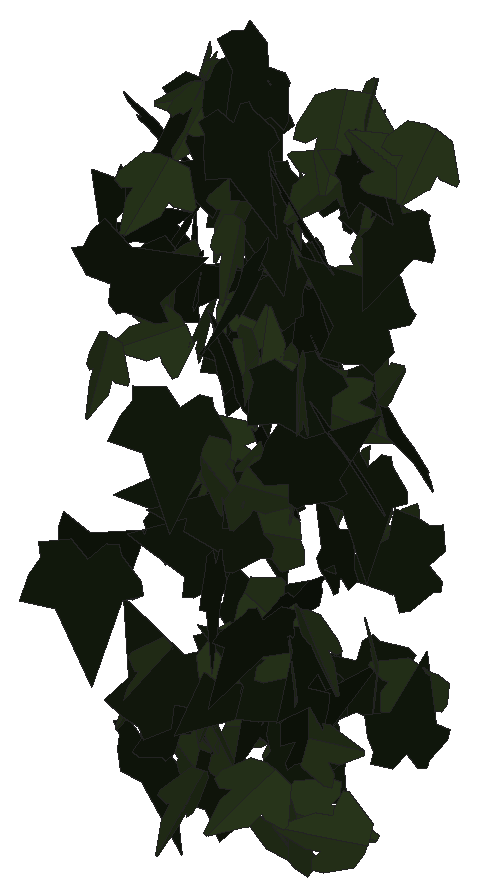
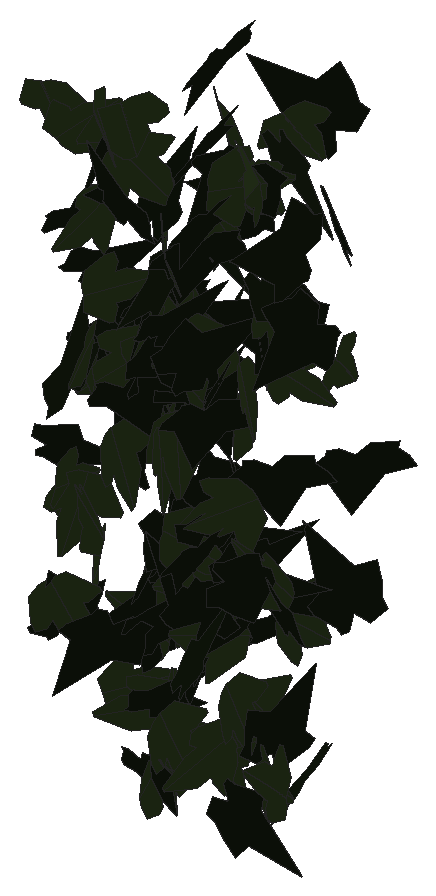
# SketchUp Ruby script. Lengths in inches.
U = 1.inch
M = Sketchup.active_model
def pt(a) = Geom::Point3d.new(a.map { |v| v * U })
def face(e, loops, mat)
  f = e.add_face(loops[0].map { |a| pt(a) })
  loops[1..].each { |l| e.add_face(l.map { |a| pt(a) }).erase! }
  f.material = f.back_material = mat if mat
  f
end
# faces: each face lists its corners as indices into pts; further lists are holes
def faces(e, pts, list, mat = nil) = list.each { |f| face(e, (f[0].is_a?(Array) ? f : [f]).map { |l| l.map { |i| pts[i] } }, mat) }
# xy, xz, yz: faces in a plane at the given z, y or x. An outline is a flat list of corners, or four numbers for a rectangle; further outlines are holes
def ring(l) = l.size == 4 ? [[l[0], l[1]], [l[2], l[1]], [l[2], l[3]], [l[0], l[3]]] : l.each_slice(2).to_a
def flat(e, list, mat, &to3) = list.each { |f| face(e, (f[0].is_a?(Array) ? f : [f]).map { |l| ring(l).map { |u, v| to3.(u, v) } }, mat) }
def xy(e, z, list, mat = nil) = flat(e, list, mat) { |x, y| [x, y, z] }
def xz(e, y, list, mat = nil) = flat(e, list, mat) { |x, z| [x, y, z] }
def yz(e, x, list, mat = nil) = flat(e, list, mat) { |y, z| [x, y, z] }
def lines(e, pts, list) = list.each { |a, b| e.add_line(pt(pts[a]), pt(pts[b])) }
# prism: a flat outline (further loops are holes) pulled along v
def prism(e, loops, v, mat = nil)
  f = face(e, loops, mat); d = Geom::Vector3d.new(v.map { |x| x * U })
  f.pushpull(f.normal.samedirection?(d) ? d.length : -d.length)
end
def box(e, o, s, mat = nil) = prism(e, [[o, [o[0] + s[0], o[1], o[2]], [o[0] + s[0], o[1] + s[1], o[2]], [o[0], o[1] + s[1], o[2]]]], [0, 0, s[2]], mat)
def at(x, y, z, deg = 0) = Geom::Transformation.translation(pt([x, y, z])) * Geom::Transformation.rotation(ORIGIN, Z_AXIS, deg.degrees)
def axes(o, x, y, z) = Geom::Transformation.new([*x, 0, *y, 0, *z, 0, *pt(o).to_a, 1])
def part(name) = M.definitions.add(name)
# library, detail: a bought-in or finely detailed component or shape, given as its bounding box
def library(name, o, s) = part(name).tap { |d| box(d.entities, o, s) }
def detail(e, o, s) = box(e.add_group.entities, o, s)
def put(e, d, t, mat = nil) = e.add_instance(d, t).tap { |i| i.material = mat if mat }
def group(e, t, mat = nil) = e.add_group.tap { |g| g.transformation = t; g.material = mat if mat }.entities
root = M.entities
M.materials.add("efeu1").color = [18, 25, 13]
M.materials.add("efeu2").color = [43, 57, 29]
c1 = part("ivyleaf_9")
p = [[1.54,2.16,1.25],[1.36,2.04,1.19],[-0.21,0.99,0.68],[-0.71,1.11,0.82],[-0.85,0.86,0.67],[-0.8,0.17,0.21],
  [-0.9,-0.01,0.1],[-0.67,-0.16,-0.02],[-0.08,-0.08,-0.05],[-0.03,-0.6,-0.4],[0.65,-0.88,-0.66],[0.83,-0.6,-0.49],
  [1.29,-0.42,-0.43],[1.8125,-0.07,-0.26],[1.21,0.44,0.15]]
faces(c1.entities,p,[[0,1,2,3,4,5,6,7,8,9,10,11,12,13,14]],"efeu1")
c2 = part("ivyleaf_10")
p = [[0,0.5,-0.03],[-0.0625,2.02,-0.43],[-0.19,2.01,-0.46],[-0.54,1.05,-0.29],[-0.52,0.625,-0.18],[-0.83,0.76,-0.28],
  [-1.16,0.64,-0.33],[-1.15,0.33,-0.24],[-0.77,-0.39,0.02],[-0.3,-0.51,0.16],[0.04,-0.48,0.23],[-0.02,2.01,-0.4375],
  [-0.06,2.01,-0.43],[0.04,-0.49,0.23],[0.67,-0.49,0.14],[1.38,0.36,-0.2],[1.375,0.51,-0.24],[0.81,0.65,-0.19],
  [0.62,0.59,-0.15],[0.6,1.09,-0.28],[0.5,1.23,-0.31]]
faces(c2.entities,p,[[0,1,2,3,4,5,6,7,8,9,10],[11,12,0,13,14,15,16,17,18,19,20]],"efeu2")
put(root,c1,axes([554.73,122.11,203.35],[0.06947,-0.03569,1.15238],[1.07212,-0.42261,-0.07772],[0.42405,1.07434,0.00771]))
put(root,c1,axes([552.73,123.43,193.32],[-0.38403,-0.96661,-0.43365],[0.17577,0.39674,-1.03999],[1.04475,-0.42206,0.01557]))
put(root,c2,axes([556.73,124.76,204.33],[0.79665,-0.51106,0.18272],[0.15582,-0.09549,-0.94648],[0.51989,0.81174,0.00369]))
put(root,c2,axes([553.95,125.07,205.125],[0.60791,0.54771,-0.47669],[-0.35161,-0.3219,-0.81825],[-0.63529,0.70226,-0.00328]))
put(root,c2,axes([559.32,124.9,193.11],[-0.83868,0.43825,-0.34025],[0.29622,-0.16775,-0.94622],[-0.46914,-0.88939,0.01081]))
put(root,c2,axes([557.21,125.36,187.27],[0.53549,0.45469,-0.69958],[-0.55938,-0.42114,-0.70188],[-0.61907,0.77383,0.02908]))
put(root,c1,axes([556.99,125.64,192.01],[-0.11361,0.57953,-0.79444],[0.18654,-0.7725,-0.5902],[-0.9655,-0.21744,-0.02055]))
put(root,c2,axes([557.96,126.16,199.61],[-0.10417,0.22538,-1.01255],[0.39339,-0.93304,-0.24815],[-0.95984,-0.40686,0.00818]))
put(root,c1,axes([556.06,125.68,207.01],[0.39115,-0.94154,-0.38299],[-0.14357,0.35508,-1.01955],[1.00627,0.41665,0.00341]))
put(root,c2,axes([551.32,126.07,198.24],[0.01117,0.68623,-0.62586],[-0.02562,-0.62544,-0.68623],[-0.92842,0.02552,0.01141]))
put(root,c2,axes([552.84,126.42,189.01],[0.14618,-0.63831,0.81545],[0.14311,-0.80318,-0.65436],[1.02563,0.20305,-0.02492]))
put(root,c2,axes([553.98,126.4,185.58],[0.13344,-0.81199,0.58918],[0.09231,-0.58191,-0.82288],[0.99897,0.16223,-0.00267]))
put(root,c1,axes([554.86,126.31,192.63],[-0.39951,0.01616,-0.88873],[0.87586,-0.15899,-0.39661],[-0.15157,-0.96134,0.05066]))
put(root,c1,axes([552,125.56,202.88],[-0.46648,0.19774,-0.78509],[-0.78387,0.11635,0.49506],[0.20253,0.90577,0.10781]))
put(root,c1,axes([553.51,126.12,188.21],[-0.67727,-0.7664,0.23334],[0.1552,0.17425,1.02277],[-0.78596,0.69482,0.00089]))
put(root,c1,axes([557.96,125.77,196.74],[-0.092,-0.05453,1.03704],[1.00297,0.26521,0.10292],[-0.2692,1.00676,0.02905]))
put(root,c1,axes([553.21,126.34,205.01],[-0.74843,0.76046,-0.04851],[0.0259,-0.04257,-1.06692],[-0.76156,-0.74879,0.01139]))
put(root,c2,axes([554.33,126.85,195.4375],[-0.128,0.06819,-0.96168],[0.74801,-0.60503,-0.14246],[-0.60825,-0.7584,0.02718]))
put(root,c2,axes([556.74,127.24,189.88],[-0.07817,0.06743,1.06056],[0.8634,-0.61598,0.1028],[0.61959,0.86688,-0.00945]))
put(root,c2,axes([556.16,126.2,195.77],[-0.29915,-0.50266,-0.84866],[0.43104,0.73105,-0.58494],[0.88718,-0.52467,-0.00197]))
put(root,c1,axes([555.7,126.99,201.82],[-0.75449,0.46546,-0.42029],[0.32926,-0.2656,-0.88522],[-0.53375,-0.8218,0.04804]))
put(root,c2,axes([556.63,127.33,190.4],[-0.06613,0.54344,0.78565],[-0.13662,-0.78482,0.53136],[0.94547,-0.07539,0.13174]))
put(root,c1,axes([549.99,127.04,190.64],[-0.23408,-0.12491,0.99895],[0.856,-0.56451,0.13],[0.52988,0.85676,0.2313]))
put(root,c1,axes([556.65,127.3,189.4],[-0.45791,-0.83133,-0.32685],[-0.16296,-0.28339,0.94908],[-0.87828,0.48601,-0.00569]))
put(root,c1,axes([557.13,127.75,190.08],[0.28866,-0.38591,-0.95824],[0.71541,-0.64305,0.47449],[-0.7452,-0.76683,0.08434]))
put(root,c2,axes([558.54,127.48,185.03],[0.14346,0.2623,0.92207],[-0.49744,-0.77663,0.29832],[0.81949,-0.51734,0.01966]))
put(root,c1,axes([558.07,127.46,197.44],[0.57222,-0.67769,0.5122],[0.3359,-0.38674,-0.88694],[0.78025,0.66349,0.00619]))
put(root,c1,axes([556.91,127.15,198.99],[-0.04282,-0.8497,-0.56476],[0.04782,0.56297,-0.85063],[1.01915,-0.06212,0.01619]))
put(root,c2,axes([557.04,127.46,196.46],[0.57739,-0.69903,0.28494],[0.18329,-0.21818,-0.90665],[0.73228,0.60578,0.00227]))
put(root,c1,axes([559.15,127.52,196.64],[-0.68801,-0.34633,-0.68097],[0.61891,0.2846,-0.77005],[0.4479,-0.92525,0.01803]))
put(root,c2,axes([556.41,127.4375,184.03],[-1.04615,0.01951,0.22966],[0.22868,-0.04542,1.04556],[0.02878,1.0701,0.04019]))
put(root,c1,axes([555.06,127.48,197.73],[0.26047,-0.80529,0.40639],[-0.05147,0.40904,0.84353],[-0.90056,-0.25629,0.06934]))
put(root,c2,axes([555.37,127.19,198.99],[0.46553,-0.54752,-0.60802],[-0.39536,0.46193,-0.71867],[0.71635,0.61076,-0.00152]))
put(root,c2,axes([557.05,127.49,187.61],[-0.28529,-0.09337,1.02708],[1.01901,0.13859,0.29565],[-0.15883,1.05692,0.05196]))
put(root,c1,axes([555.53,127.98,195.23],[0.21586,-0.30888,0.92443],[0.48939,-0.78447,-0.37639],[0.84289,0.53457,-0.0182]))
put(root,c1,axes([554.32,128.39,188.39],[-0.42195,-0.70639,0.65777],[-0.29008,-0.59189,-0.82171],[0.9206,-0.51027,0.04257]))
put(root,c1,axes([556.45,127.67,191.65],[-0.30841,0.77516,-0.55379],[0.20481,-0.51452,-0.83426],[-0.93038,-0.37022,-0.00008]))
put(root,c2,axes([552.08,127.78,198.4375],[0.47091,0.07208,-0.78678],[-0.78456,-0.06543,-0.47557],[-0.09324,0.9146,0.02799]))
put(root,c2,axes([555.47,127.54,198.36],[0.94538,0.10195,-0.02577],[0.02549,0.00397,0.95086],[0.10202,-0.94572,0.00121]))
put(root,c2,axes([552.26,127.68,200.62],[-0.24424,-1.03607,-0.08668],[0.01125,0.0864,-1.06443],[1.03963,-0.24434,-0.00884]))
put(root,c1,axes([554.89,128.32,187.98],[0.00004,-0.00768,-0.94566],[0.70171,-0.63397,0.00518],[-0.63399,-0.70168,0.00567]))
put(root,c2,axes([554.11,128.34,203.17],[0.05469,-0.78668,0.55718],[0.20089,-0.53653,-0.77724],[0.94285,0.15995,0.13328]))
put(root,c1,axes([553.08,127.76,204.02],[0.35461,-0.03639,-0.85389],[0.72281,0.5061,0.2786],[0.45608,-0.77379,0.22238]))
put(root,c1,axes([558.16,127.54,193.2],[0.19785,-0.16216,0.92337],[-0.43001,0.82289,0.23665],[-0.83307,-0.46327,0.09715]))
put(root,c2,axes([556.75,127.61,185.23],[-0.29659,-0.13942,-1.02034],[0.99377,0.23974,-0.32162],[0.2701,-1.03517,0.06294]))
put(root,c1,axes([551.97,128.34,185.72],[0.25084,0.30872,0.88717],[-0.69039,-0.56208,0.3908],[0.63697,-0.73079,0.0742]))
put(root,c1,axes([550.88,128.26,184.96],[0.50801,-0.9688,0.10046],[0.05093,-0.08672,-1.0939],[0.97266,0.51053,0.00481]))
put(root,c1,axes([551.61,127.68,199.69],[0.39481,0.00406,1.03661],[1.03638,-0.02493,-0.39462],[0.02186,1.10896,-0.01267]))
put(root,c1,axes([557.08,127.15,187.84],[0.14985,0.25189,1.10714],[0.58147,0.94216,-0.29306],[-0.97524,0.60045,-0.00462]))
put(root,c1,axes([553.04,128.83,191.46],[-0.17736,-0.07382,1.03308],[-0.79743,-0.65909,-0.184],[0.66091,-0.81505,0.05523]))
put(root,c1,axes([551.82,128.52,195.46],[-0.54493,-0.88274,-0.40095],[0.22315,0.3334,-1.0373],[0.9435,-0.58869,0.01376]))
put(root,c1,axes([556.41,128.45,202.52],[0.5722,-0.74475,0.46475],[-0.26041,0.38579,0.93883],[-0.83835,-0.62814,0.02558]))
put(root,c2,axes([558.46,128.68,189.82],[-0.34485,0.25719,0.93352],[0.75402,-0.55039,0.43018],[0.6075,0.82913,-0.00401]))
put(root,c2,axes([555.98,128.44,197.53],[-0.67706,-0.9214,-0.03429],[-0.00294,-0.04039,1.14321],[-0.92203,0.67672,0.02153]))
put(root,c2,axes([554.05,127.56,188.5],[0.23066,0.19503,-1.08225],[0.65803,0.86149,0.2955],[0.88107,-0.69447,0.06264]))
put(root,c1,axes([556.62,129.04,188.28],[-0.42272,-0.31573,0.75062],[-0.55364,-0.50875,-0.52579],[0.59715,-0.69519,0.04388]))
put(root,c2,axes([554.59,128.41,190.49],[0.33594,0.09789,0.93206],[0.9051,0.22299,-0.34964],[-0.24314,0.96534,-0.01375]))
put(root,c1,axes([552.24,128.48,201.55],[-0.58376,0.68743,-0.20394],[0.13213,-0.15535,-0.90186],[-0.70477,-0.59853,-0.00015]))
put(root,c1,axes([560.07,128.85,193.51],[-0.67677,-0.01452,0.65017],[-0.64847,-0.05571,-0.67625],[0.04906,-0.93682,0.03014]))
put(root,c2,axes([552.48,128.9,205.15],[0.34214,0.6651,-0.58723],[-0.31652,-0.49647,-0.74672],[-0.82886,0.46413,0.04275]))
put(root,c2,axes([557.02,129.05,204.49],[-0.44709,-0.61172,0.73961],[-0.43524,-0.59798,-0.75769],[0.85545,-0.62396,0.00104]))
put(root,c1,axes([556.47,128.2,200.17],[0.3827,-0.26813,-0.83036],[-0.66452,0.49808,-0.4671],[0.56551,0.76674,0.01305]))
put(root,c1,axes([554.3,128.73,189.375],[-0.31888,0.14608,1.05736],[0.87617,-0.59447,0.34637],[0.60966,0.93075,0.05527]))
put(root,c2,axes([555.34,128.73,195.65],[-0.37249,-0.96651,-0.04003],[0.01408,0.03748,-1.03581],[0.96724,-0.37276,-0.00034]))
put(root,c1,axes([554.41,128.69,198.33],[0.35645,0.698,-0.69959],[-0.32915,-0.61739,-0.78369],[-0.93182,0.48509,0.00921]))
put(root,c1,axes([556.17,128.87,185.93],[-0.65703,-0.63451,-0.00932],[-0.00576,-0.00745,0.9134],[-0.63455,0.65706,0.00135]))
put(root,c2,axes([552.85,129.11,187.43],[0.10522,-0.96606,0.26786],[0.03889,-0.2652,-0.97173],[1.00176,0.11177,0.00959]))
put(root,c1,axes([553.5,128.59,198.33],[0.53168,-0.55021,-0.5356],[-0.35282,0.40357,-0.76481],[0.682,0.63772,0.02189]))
put(root,c1,axes([553.99,129.27,192.4],[-0.4768,-0.03955,0.92066],[-0.8904,-0.24732,-0.47175],[0.23744,-1.00687,0.07972]))
put(root,c2,axes([556.94,128.375,197.52],[-0.56879,-0.29266,-0.91905],[0.79513,0.46167,-0.6391],[0.54596,-0.97726,-0.02669]))
put(root,c1,axes([558.44,129.11,200.19],[-0.66642,-0.74334,-0.28833],[-0.19769,-0.21001,0.99832],[-0.77241,0.69509,-0.00673]))
put(root,c2,axes([553.45,128.5625,185.23],[-0.41649,0.31669,-0.77791],[-0.61672,0.47414,0.52321],[0.57017,0.74418,-0.00231]))
put(root,c2,axes([552.04,128.73,184.79],[0.17219,-0.05341,0.90413],[-0.88798,0.17123,0.17922],[-0.1783,-0.90431,-0.01946]))
put(root,c1,axes([550.32,128.47,200.86],[0.6947,0.55374,0.20711],[0.16395,0.12659,-0.88838],[-0.56801,0.71378,-0.00312]))
put(root,c1,axes([550.22,129.16,203.65],[0.83035,-0.52072,0.48441],[0.41775,-0.24554,-0.98004],[0.57558,0.92943,0.01248]))
put(root,c2,axes([552.77,129.65,205.28],[0.02352,0.06694,-1.05229],[-0.77478,-0.71285,-0.06266],[-0.71521,0.77442,0.03328]))
put(root,c1,axes([559.55,128.73,187.66],[-0.45807,-0.38586,0.69445],[0.52612,0.4533,0.5989],[-0.59527,0.69757,-0.00506]))
put(root,c1,axes([552.26,128.57,199.27],[0.13673,-0.08442,0.91084],[-0.13704,0.90868,0.10479],[-0.90442,-0.15045,0.12182]))
put(root,c1,axes([553.7,129.96,206.14],[-0.17416,-0.8045,0.71653],[-0.07965,-0.71423,-0.82128],[1.07438,-0.18336,0.05526]))
put(root,c1,axes([557.64,128.83,205.25],[0.42606,-0.45107,-0.65872],[-0.46043,0.47115,-0.62042],[0.65222,0.62726,-0.00767]))
put(root,c2,axes([552.37,129.2,198.63],[0.33931,-0.87683,-0.10025],[-0.02016,0.09968,-0.94004],[0.88232,0.33947,0.01708]))
put(root,c1,axes([558.52,129.82,196.57],[0.83104,-0.52748,-0.44182],[0.39373,-0.20361,0.98366],[-0.56428,-0.9189,0.03566]))
put(root,c2,axes([556.87,129.32,206.2],[0.65026,0.89956,-0.27856],[-0.18434,-0.21038,-1.10968],[-0.92348,0.6754,0.02537]))
put(root,c2,axes([558.86,129.47,204.94],[0.40261,0.49015,0.7051],[-0.46929,-0.52658,0.63402],[0.71915,-0.61804,0.01899]))
put(root,c2,axes([553.94,129.49,197.75],[-0.15328,-0.01895,1.02335],[1.00957,-0.1731,0.14801],[0.16846,1.02018,0.04412]))
put(root,c1,axes([552.56,129.02,205.67],[-0.23469,-0.38765,-0.94717],[0.41761,0.8509,-0.45172],[0.93435,-0.47768,-0.03601]))
put(root,c2,axes([554.83,129.42,192.32],[-0.14826,-0.02139,1.06528],[-1.02151,-0.30301,-0.14825],[0.30301,-1.03199,0.02145]))
put(root,c1,axes([553.85,129.57,202.81],[-0.15719,-0.92378,-0.4774],[0.11293,0.4648,-0.93658],[1.03369,-0.19125,0.02973]))
put(root,c1,axes([555.59,130.23,198.13],[-0.19143,-0.24057,0.98515],[-0.47433,-0.86488,-0.30337],[0.89632,-0.50907,0.04986]))
put(root,c2,axes([559.59,129.53,206.05],[0.92798,0.06573,-0.25854],[-0.25903,-0.00163,-0.93016],[-0.06376,0.96332,0.01606]))
put(root,c2,axes([555.42,129.32,195.38],[0.24295,-0.93196,-0.3254],[-0.0358,0.32657,-0.96204],[0.98648,0.24137,0.04522]))
put(root,c2,axes([556.86,129.67,195.01],[0.0638,-1.03745,0.12459],[0.00306,-0.12463,-1.0394],[1.0449,0.06371,-0.00457]))
put(root,c2,axes([555.44,128.97,184.24],[-0.05649,0.1057,-0.9716],[-0.6434,0.72856,0.11667],[0.73568,0.64529,0.02743]))
put(root,c1,axes([550.62,129.39,190.88],[-0.35986,0.53399,0.64734],[0.38316,-0.52209,0.64367],[0.74658,0.52534,-0.01832]))
put(root,c2,axes([550.64,129.68,185.29],[-0.00082,-0.2175,0.94094],[0.9585,-0.11521,-0.0258],[0.11806,0.93386,0.21596]))
put(root,c2,axes([553.51,129.03,199.15],[0.23249,0.16499,0.98686],[0.71344,0.68301,-0.28227],[-0.70152,0.7493,0.04]))
put(root,c1,axes([552.62,129.53,184.09],[-0.08065,-0.02592,-1.05543],[-0.93515,-0.48951,0.08348],[-0.48998,0.93851,0.0144]))
put(root,c2,axes([552.39,129.35,194.37],[-0.55869,-0.11437,-0.87816],[0.87925,0.05224,-0.56619],[0.10565,-1.0395,0.06816]))
put(root,c2,axes([552.13,128.98,205.24],[0.37952,-0.12595,0.85868],[-0.5765,0.66396,0.35219],[-0.64872,-0.66372,0.18937]))
put(root,c2,axes([550.67,129.72,192.31],[0.39882,-0.19884,-0.90022],[0.86631,-0.25468,0.44005],[-0.31535,-0.95111,0.07037]))
put(root,c2,axes([559.08,129.84,189.17],[-0.66399,-0.45428,0.51951],[-0.40068,-0.3332,-0.80348],[0.56188,-0.77444,0.04095]))
put(root,c2,axes([554.58,130.13,202.36],[0.47535,-0.25127,0.8398],[0.70964,-0.45052,-0.53647],[0.5146,0.85338,-0.03595]))
put(root,c1,axes([558.09,130.27,202.95],[-0.40489,-0.86177,0.12051],[-0.03237,-0.11791,-0.95193],[0.86956,-0.40566,0.02068]))
put(root,c2,axes([558.45,130.3125,193.41],[0.01996,0.20091,-0.85382],[-0.17587,-0.83578,-0.20077],[-0.85933,0.17572,0.02126]))
put(root,c1,axes([554.96,129.98,199.625],[-0.51644,-0.87799,-0.04218],[-0.01445,-0.04044,1.01859],[-0.87889,0.51658,0.00804]))
put(root,c2,axes([555.08,130.41,184.18],[-0.07562,0.1182,1.04111],[0.59139,-0.85686,0.14023],[0.86496,0.59618,-0.00486]))
put(root,c2,axes([554.59,130.09,186.27],[-0.06391,-0.95484,0.36693],[-0.00709,-0.36722,-0.95684],[1.02289,-0.06221,0.01629]))
put(root,c1,axes([556.12,130.1875,197.4],[-0.70109,-0.74002,-0.23058],[0.16187,0.16426,-1.01938],[0.75802,-0.71952,0.00443]))
put(root,c1,axes([555.02,129.69,201.4],[0.78278,-0.40489,-0.12318],[-0.10891,0.05755,-0.88129],[0.40895,0.79032,0.00107]))
put(root,c2,axes([557.05,130.22,206.29],[0.66472,-0.68417,0.48045],[0.33179,-0.34751,-0.9539],[0.76736,0.74292,-0.00374]))
put(root,c1,axes([552.04,130.38,192.3],[-0.28584,-0.45618,-0.90021],[-0.41433,-0.80009,0.53701],[-0.92022,0.50194,0.03784]))
put(root,c1,axes([553.79,130.5,199.01],[-0.12527,-0.07301,1.05439],[-0.87631,-0.58643,-0.14472],[0.59089,-0.88518,0.00891]))
put(root,c2,axes([556.97,130.5,200.64],[-0.04764,-0.01804,-0.91004],[-0.6402,-0.64713,0.04634],[-0.64703,0.64162,0.02115]))
put(root,c1,axes([553.39,130.15,192.89],[0.13721,-0.88823,-0.26019],[-0.00155,0.26282,-0.898],[0.92556,0.13212,0.03707]))
put(root,c2,axes([558.12,129.73,193.06],[-0.51168,-0.80094,-0.39216],[0.22066,0.32436,-0.95037],[0.86406,-0.55714,0.01047]))
put(root,c1,axes([553.15,130.15,197.625],[-0.28563,-0.79043,-0.46824],[0.13397,0.44927,-0.84013],[0.90888,-0.31462,-0.02331]))
put(root,c1,axes([556.4375,129.78,203.01],[-0.65425,0.53903,0.58756],[0.4309,-0.40048,0.84721],[0.6709,0.78287,0.02883]))
put(root,c1,axes([553.71,130.41,188.43],[0.38853,-0.90706,0.23078],[-0.08177,0.21602,0.98673],[-0.93238,-0.39692,0.00963]))
put(root,c1,axes([555.31,130.39,185.02],[-0.80605,-0.19675,-0.30461],[0.29453,0.07791,-0.8297],[0.21155,-0.85816,-0.00548]))
put(root,c2,axes([557.08,130.55,192.49],[0.23141,-0.21025,-0.99383],[0.74754,-0.65492,0.31261],[-0.68782,-0.78252,0.00539]))
put(root,c2,axes([553.14,129.46,185.89],[-0.16451,-0.38781,-0.99947],[0.44798,0.89379,-0.42054],[0.97398,-0.4766,0.02461]))
put(root,c1,axes([553.01,130.25,204.42],[0.19814,-0.83427,-0.33473],[-0.07643,0.32589,-0.85748],[0.89566,0.21236,0.00088]))
put(root,c2,axes([558.04,129.47,197.85],[0.07779,-0.18076,-0.96008],[-0.11389,0.95487,-0.18901],[0.97028,0.12657,0.05479]))
put(root,c1,axes([556.93,129.92,188.84],[-0.03918,-0.50955,-0.87742],[0.11169,0.87058,-0.51056],[1.00848,-0.11621,0.02246]))
put(root,c2,axes([557.62,129.6,202.84],[-0.09201,-0.36241,-0.93936],[0.30744,0.88811,-0.37276],[0.95876,-0.31957,0.02938]))
